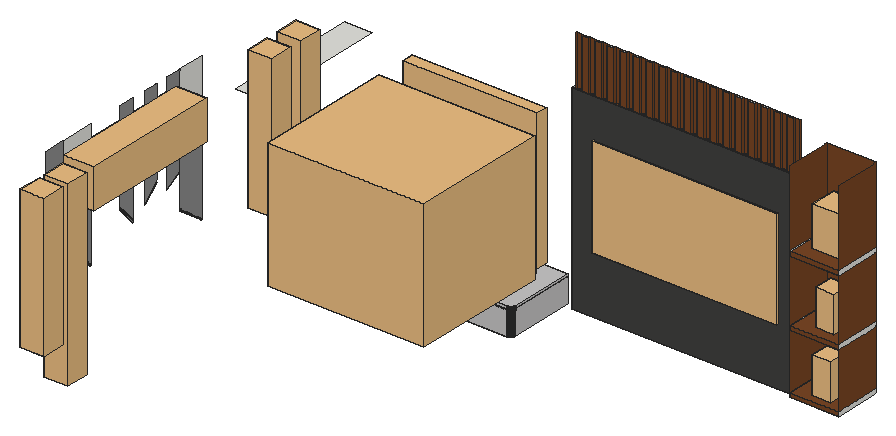
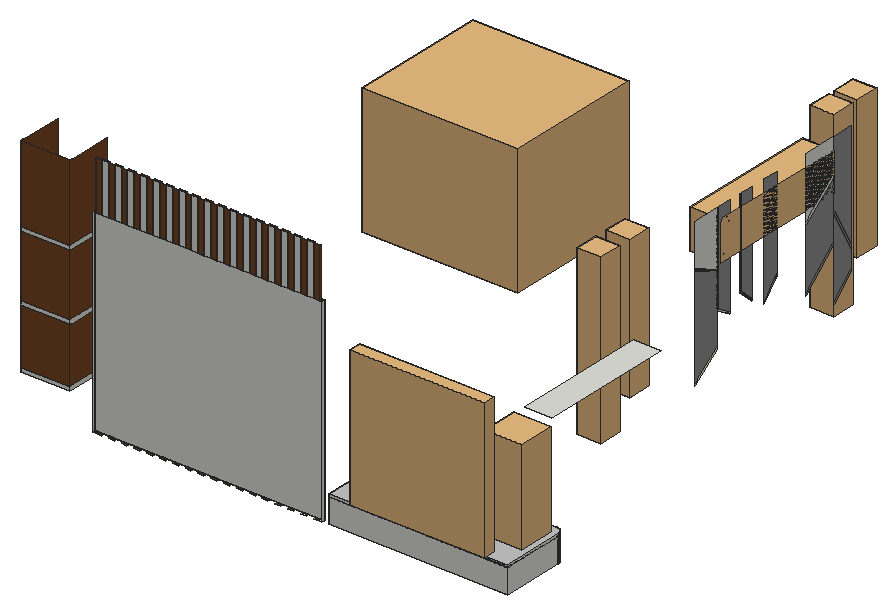
# SketchUp Ruby script. Lengths in inches.
U = 1.inch
M = Sketchup.active_model
def pt(a) = Geom::Point3d.new(a.map { |v| v * U })
def face(e, loops, mat)
  f = e.add_face(loops[0].map { |a| pt(a) })
  loops[1..].each { |l| e.add_face(l.map { |a| pt(a) }).erase! }
  f.material = f.back_material = mat if mat
  f
end
# faces: each face lists its corners as indices into pts; further lists are holes
def faces(e, pts, list, mat = nil) = list.each { |f| face(e, (f[0].is_a?(Array) ? f : [f]).map { |l| l.map { |i| pts[i] } }, mat) }
# xy, xz, yz: faces in a plane at the given z, y or x. An outline is a flat list of corners, or four numbers for a rectangle; further outlines are holes
def ring(l) = l.size == 4 ? [[l[0], l[1]], [l[2], l[1]], [l[2], l[3]], [l[0], l[3]]] : l.each_slice(2).to_a
def flat(e, list, mat, &to3) = list.each { |f| face(e, (f[0].is_a?(Array) ? f : [f]).map { |l| ring(l).map { |u, v| to3.(u, v) } }, mat) }
def xy(e, z, list, mat = nil) = flat(e, list, mat) { |x, y| [x, y, z] }
def xz(e, y, list, mat = nil) = flat(e, list, mat) { |x, z| [x, y, z] }
def yz(e, x, list, mat = nil) = flat(e, list, mat) { |y, z| [x, y, z] }
def lines(e, pts, list) = list.each { |a, b| e.add_line(pt(pts[a]), pt(pts[b])) }
# prism: a flat outline (further loops are holes) pulled along v
def prism(e, loops, v, mat = nil)
  f = face(e, loops, mat); d = Geom::Vector3d.new(v.map { |x| x * U })
  f.pushpull(f.normal.samedirection?(d) ? d.length : -d.length)
end
def box(e, o, s, mat = nil) = prism(e, [[o, [o[0] + s[0], o[1], o[2]], [o[0] + s[0], o[1] + s[1], o[2]], [o[0], o[1] + s[1], o[2]]]], [0, 0, s[2]], mat)
def at(x, y, z, deg = 0) = Geom::Transformation.translation(pt([x, y, z])) * Geom::Transformation.rotation(ORIGIN, Z_AXIS, deg.degrees)
def axes(o, x, y, z) = Geom::Transformation.new([*x, 0, *y, 0, *z, 0, *pt(o).to_a, 1])
def part(name) = M.definitions.add(name)
# library, detail: a bought-in or finely detailed component or shape, given as its bounding box
def library(name, o, s) = part(name).tap { |d| box(d.entities, o, s) }
def detail(e, o, s) = box(e.add_group.entities, o, s)
def put(e, d, t, mat = nil) = e.add_instance(d, t).tap { |i| i.material = mat if mat }
def group(e, t, mat = nil) = e.add_group.tap { |g| g.transformation = t; g.material = mat if mat }.entities
root = M.entities
M.materials.add("Emissive").color = [234, 236, 196]
M.materials.add("Generic").color = [198, 197, 197]
M.materials.add("Gold 10k").color = [251, 232, 180]
M.materials.add("Magma Rock Solid 19-50 100cm").color = [65, 65, 64]
M.materials.add("[Color M04]").color = [142, 142, 142]
M.materials.add("[Wood Veneer 01]").color = [120, 70, 37]
c1 = library("Lady Jane Collar",[-41.56,-7.87,0],[83.12,15.74,85.88])
c2 = library("Flowering Tree Twigs 63-18",[-6.76,-5.61,0],[12.33,12.14,31.28])
c3 = library("Milk Jug 92-17",[-1.54,-2.02,0],[3.08,4.6,8.29])
c4 = library("Vase Gerbera 18",[-3.31,-2.98,0],[6.3,6.31,11.9375])
c5 = library("Flat screen television",[0,1.41,1.14],[35.92,0.28,20.21])
c6 = library("Pendant 114-23",[-3.9375,-3.9375,-46.79],[7.875,7.875,46.79])
c7 = library("Milk Jug 92-23",[-3.1,-3.1,0],[6.18,6.2,11.88])
c8 = library("CUONGCV (3)",[45.61,64.16,23.25],[51.6,45.8,42.59])
c9 = library("Calla Lilies 63-10",[-4.34,-4.49,0],[8.67,8.83,13.09])
c10 = library("Streamline AC Unit ",[11.33,77.43,-2],[10.25,46.46,12.99])
xy(root,38.375,[[17.14,344.6875,16.8,344.71,16.46,344.78,16.13,344.89,15.82,345.04,15.53,345.23,15.27,345.46,15.05,345.72,14.85,346.01,14.7,346.32,14.59,346.64,14.52,346.98,14.5,347.33,14.5,367.875,73.93,367.875,73.93,346.37,73.91,346.15,73.87,345.93,73.8,345.72,73.7,345.53,73.58,345.34,73.43,345.18,73.27,345.03,73.09,344.91,72.89,344.82,72.68,344.74,72.47,344.7,72.25,344.6875],[150.92,366.625,151.83,367],[76.01,367.25,76.95,367.875],[76.95,367.25,78.89,367.875],[81.19,367.25,83.125,367.875],
  [150.92,367.25,151.83,367.875]])
xy(root,38.375,[[76.01,366.625,150.92,367]],"Magma Rock Solid 19-50 100cm")
xy(root,38.375,[[150.92,367,151.58,367.25],[85.43,367.25,87.36,367.875],[89.67,367.25,91.6,367.875],[93.9,367.25,95.84,367.875],[98.14,367.25,100.07,367.875],
  [102.38,367.25,104.3125,367.875],[106.62,367.25,108.55,367.875],[110.85,367.25,112.79,367.875],[115.09,367.25,117.02,367.875],[119.33,367.25,121.26,367.875],
  [123.57,367.25,125.5,367.875],[127.8,367.25,129.74,367.875],[132.04,367.25,133.97,367.875],[136.28,367.25,138.21,367.875],[140.52,367.25,142.45,367.875],
  [144.75,367.25,146.6875,367.875],[148.99,367.25,150.92,367.875]],"[Wood Veneer 01]")
xy(root,38.625,[[76.26,367,150.92,367.25]],"Emissive")
xy(root,46.375,[[17.14,344.6875,16.8,344.71,16.46,344.78,16.13,344.89,15.82,345.04,15.53,345.23,15.27,345.46,15.05,345.72,14.85,346.01,14.7,346.32,14.59,346.64,14.52,346.98,14.5,347.33,14.5,367.875,73.93,367.875,73.93,346.37,73.91,346.15,73.87,345.93,73.8,345.72,73.7,345.53,73.58,345.34,73.43,345.18,73.27,345.03,73.09,344.91,72.89,344.82,72.68,344.74,72.47,344.7,72.25,344.6875]])
xy(root,46.625,[[17.14,344.6875,16.8,344.71,16.46,344.78,16.13,344.89,15.82,345.04,15.53,345.23,15.27,345.46,15.05,345.72,14.85,346.01,14.7,346.32,14.59,346.64,14.52,346.98,14.5,347.33,14.5,367.875,73.93,367.875,73.93,346.37,73.91,346.15,73.87,345.93,73.8,345.72,73.7,345.53,73.58,345.34,73.43,345.18,73.27,345.03,73.09,344.91,72.89,344.82,72.68,344.74,72.47,344.7,72.25,344.6875]])
xy(root,47.375,[[17.14,344.6875,72.25,344.6875,72.47,344.7,72.68,344.74,72.89,344.82,73.09,344.91,73.27,345.03,73.43,345.18,73.58,345.34,73.7,345.53,73.8,345.72,73.87,345.93,73.91,346.15,73.93,346.37,73.93,367.875,14.5,367.875,14.5,347.33,14.52,346.98,14.59,346.64,14.7,346.32,14.85,346.01,15.05,345.72,15.27,345.46,15.53,345.23,15.82,345.04,16.13,344.89,16.46,344.78,16.8,344.71]],"Generic")
xy(root,47.59,[[159.58,352.5625,175.89,366.875]],"[Wood Veneer 01]")
xy(root,47.84,[[159.58,366.875,175.89,367.875]],"Emissive")
xy(root,48.99,[[159.58,352.5625,175.89,367.875]],"[Wood Veneer 01]")
xy(root,67.4,[[159.58,352.5625,175.89,366.875]],"[Wood Veneer 01]")
xy(root,67.65,[[159.58,366.875,175.89,367.875]],"Emissive")
xy(root,68.8,[[159.58,352.5625,175.89,367.875]],"[Wood Veneer 01]")
xy(root,89.4,[[159.58,352.5625,175.89,366.875]],"[Wood Veneer 01]")
xy(root,89.65,[[159.58,366.875,175.89,367.875]],"Emissive")
xy(root,90.8,[[159.58,352.5625,175.89,367.875]],"[Wood Veneer 01]")
xy(root,96,[[0,322.76,9,367.875]])
xy(root,103.375,[[76.26,367,151.58,367.25]],"Emissive")
xy(root,103.625,[[76.01,367.25,76.95,367.875],[78.89,367.25,81.19,367.875],[83.125,367.25,85.43,367.875],[87.36,367.25,89.67,367.875],[91.6,367.25,93.9,367.875],
  [95.84,367.25,98.14,367.875],[100.07,367.25,102.38,367.875],[104.3125,367.25,106.62,367.875],[108.55,367.25,110.85,367.875],[112.79,367.25,115.09,367.875],
  [117.02,367.25,119.33,367.875],[121.26,367.25,123.57,367.875],[125.5,367.25,127.8,367.875],[129.74,367.25,132.04,367.875],[133.97,367.25,136.28,367.875],
  [138.21,367.25,140.52,367.875],[142.45,367.25,144.75,367.875],[146.6875,367.25,148.99,367.875],[150.92,367.25,151.83,367.875]])
xy(root,103.625,[[76.01,366.625,151.83,367]],"Magma Rock Solid 19-50 100cm")
xy(root,103.625,[[76.95,367.25,78.89,367.875],[81.19,367.25,83.125,367.875],[85.43,367.25,87.36,367.875],[89.67,367.25,91.6,367.875],[93.9,367.25,95.84,367.875],
  [98.14,367.25,100.07,367.875],[102.38,367.25,104.3125,367.875],[106.62,367.25,108.55,367.875],[110.85,367.25,112.79,367.875],[115.09,367.25,117.02,367.875],
  [119.33,367.25,121.26,367.875],[123.57,367.25,125.5,367.875],[127.8,367.25,129.74,367.875],[132.04,367.25,133.97,367.875],[136.28,367.25,138.21,367.875],
  [140.52,367.25,142.45,367.875],[144.75,367.25,146.6875,367.875],[148.99,367.25,150.92,367.875]],"[Wood Veneer 01]")
xz(root,240.18,[[8.9375,70.9375,9,97.25],[8.9375,98.25,9,120]])
xz(root,240.43,[[8.9375,88.44,9,107.62]],"[Color M04]")
xz(root,251.56,[[8.9375,99.77,9,120]])
xz(root,251.56,[[8.9375,78.66,9,99.01]],"[Color M04]")
xz(root,263.87,[[8.9375,89.91,9,120]])
xz(root,268.93,[[8.9375,83.81,9,120]],"[Color M04]")
xz(root,274.12,[[8.9375,86.8125,9,120]],"[Color M04]")
xz(root,278.81,[[8.9375,91.37,9,120]],"[Color M04]")
xz(root,283.12,[[8.9375,87,9,120]],"[Color M04]")
xz(root,288.31,[[8.9375,90.1,9,120]],"[Color M04]")
xz(root,288.56,[[8.9375,101.89,9,120]])
xz(root,288.56,[[8.9375,78.64,9,101.51]],"[Color M04]")
xz(root,344.6875,[[17.14,38.375,44.69,46.375],[45.09,38.375,72.25,46.375],[17.14,46.625,72.25,47.375]],"Generic")
xz(root,344.6875,[[44.69,38.375,45.09,46.375],[17.14,46.375,72.25,46.625]],"Gold 10k")
xz(root,352.5625,[[159.58,47.59,175.89,48.99],[159.58,67.4,175.89,68.8],[159.58,89.4,175.89,90.8]],"[Wood Veneer 01]")
xz(root,366.625,[[76.01,38.375,151.83,103.625]],"Magma Rock Solid 19-50 100cm")
xz(root,366.875,[[159.58,47.59,175.89,47.84],[159.58,67.4,175.89,67.65],[159.58,89.4,175.89,89.4375],[159.58,89.4375,175.89,89.65]],"Emissive")
xz(root,367,[[150.92,38.375,150.92,38.625,76.26,38.625,76.26,103.375,151.58,103.375,151.58,38.375]])
xz(root,367,[[76.01,38.375,150.92,38.625],[151.58,38.375,151.83,103.625],[76.01,38.625,76.26,103.375],[76.01,103.375,151.58,103.625]],"Emissive")
xz(root,367.25,[[150.92,38.375,150.92,38.625,76.26,38.625,76.26,103.375,151.58,103.375,151.58,38.375]])
xz(root,367.25,[[76.01,38.375,76.95,38.625],[76.95,38.375,78.89,38.625],[81.19,38.375,83.125,38.625],[85.43,38.375,87.36,38.625],[89.67,38.375,91.6,38.625],
  [93.9,38.375,95.84,38.625],[98.14,38.375,100.07,38.625],[102.38,38.375,104.3125,38.625],[106.62,38.375,108.55,38.625],[110.85,38.375,112.79,38.625],
  [115.09,38.375,117.02,38.625],[119.33,38.375,121.26,38.625],[123.57,38.375,125.5,38.625],[127.8,38.375,129.74,38.625],[132.04,38.375,133.97,38.625],
  [136.28,38.375,138.21,38.625],[140.52,38.375,142.45,38.625],[144.75,38.375,146.6875,38.625],[148.99,38.375,150.92,38.625],[151.58,38.375,151.83,103.625],
  [76.01,38.625,76.26,103.375],[76.01,103.375,76.95,103.625],[76.95,103.375,78.89,103.625],[78.89,103.375,81.19,103.625],[81.19,103.375,83.125,103.625],
  [83.125,103.375,85.43,103.625],[85.43,103.375,87.36,103.625],[87.36,103.375,89.67,103.625],[89.67,103.375,91.6,103.625],[91.6,103.375,93.9,103.625],
  [93.9,103.375,95.84,103.625],[95.84,103.375,98.14,103.625],[98.14,103.375,100.07,103.625],[100.07,103.375,102.38,103.625],[102.38,103.375,104.3125,103.625],
  [104.3125,103.375,106.62,103.625],[106.62,103.375,108.55,103.625],[108.55,103.375,110.85,103.625],[110.85,103.375,112.79,103.625],[112.79,103.375,115.09,103.625],
  [115.09,103.375,117.02,103.625],[117.02,103.375,119.33,103.625],[119.33,103.375,121.26,103.625],[121.26,103.375,123.57,103.625],[123.57,103.375,125.5,103.625],
  [125.5,103.375,127.8,103.625],[127.8,103.375,129.74,103.625],[129.74,103.375,132.04,103.625],[132.04,103.375,133.97,103.625],[133.97,103.375,136.28,103.625],
  [136.28,103.375,138.21,103.625],[138.21,103.375,140.52,103.625],[140.52,103.375,142.45,103.625],[142.45,103.375,144.75,103.625],[144.75,103.375,146.6875,103.625],
  [146.6875,103.375,148.99,103.625],[148.99,103.375,150.92,103.625],[150.92,103.375,151.58,103.625]],"Emissive")
xz(root,367.25,[[78.89,103.625,81.19,120],[83.125,103.625,85.43,120],[87.36,103.625,89.67,120],[91.6,103.625,93.9,120],[95.84,103.625,98.14,120],
  [100.07,103.625,102.38,120],[104.3125,103.625,106.62,120],[108.55,103.625,110.85,120],[112.79,103.625,115.09,120],[117.02,103.625,119.33,120],
  [121.26,103.625,123.57,120],[125.5,103.625,127.8,120],[129.74,103.625,132.04,120],[133.97,103.625,136.28,120],[138.21,103.625,140.52,120],
  [142.45,103.625,144.75,120],[146.6875,103.625,148.99,120]],"[Wood Veneer 01]")
xz(root,367.875,[[14.5,38.375,73.93,46.375],[14.5,46.375,73.93,46.625],[14.5,46.625,73.93,47.375],[159.58,47.84,175.89,48.99],[159.58,67.65,175.89,68.8],
  [159.58,89.65,175.89,90.8],[78.89,103.625,81.19,120],[83.125,103.625,85.43,120],[87.36,103.625,89.67,120],[91.6,103.625,93.9,120],
  [95.84,103.625,98.14,120],[100.07,103.625,102.38,120],[104.3125,103.625,106.62,120],[108.55,103.625,110.85,120],[112.79,103.625,115.09,120],
  [117.02,103.625,119.33,120],[121.26,103.625,123.57,120],[125.5,103.625,127.8,120],[129.74,103.625,132.04,120],[133.97,103.625,136.28,120],
  [138.21,103.625,140.52,120],[142.45,103.625,144.75,120],[146.6875,103.625,148.99,120]])
xz(root,367.875,[[159.58,48.99,175.89,67.65],[159.58,68.8,175.89,89.65],[159.58,90.8,175.89,116.25],[76.95,103.625,78.89,120],[81.19,103.625,83.125,120],
  [85.43,103.625,87.36,120],[89.67,103.625,91.6,120],[93.9,103.625,95.84,120],[98.14,103.625,100.07,120],[102.38,103.625,104.3125,120],
  [106.62,103.625,108.55,120],[110.85,103.625,112.79,120],[115.09,103.625,117.02,120],[119.33,103.625,121.26,120],[123.57,103.625,125.5,120],
  [127.8,103.625,129.74,120],[132.04,103.625,133.97,120],[136.28,103.625,138.21,120],[140.52,103.625,142.45,120],[144.75,103.625,146.6875,120],
  [148.99,103.625,150.92,120]],"[Wood Veneer 01]")
yz(root,8.9375,[[251.56,99.01,251.56,99.77,240.43,108.38,240.43,107.62]])
yz(root,8.9375,[[297.48,71.32,297.48,71.82,288.56,78.64,288.56,78.14],[283.12,86.5,288.31,89.6,288.31,90.1,283.12,87],[288.56,101.51,297.48,105.77,297.48,106.14,288.56,101.89]],"Emissive")
yz(root,8.9375,[[240.18,70.25,240.18,70.9375,233,77.53,233,76.84],[251.56,77.93,251.56,78.66,240.43,88.44,240.43,87.71],[268.93,83.18,268.93,83.81,263.87,89.91,263.87,89.29],[233,83.85,240.18,97.25,240.18,98.25,233,84.85],[274.12,86.125,278.81,90.68,278.81,91.37,274.12,86.8125]],"[Color M04]")
yz(root,9,[[251.56,99.77,251.56,120,240.43,120,240.43,108.38],[288.56,101.89,297.48,106.14,297.48,120,288.56,120]])
yz(root,9,[[240.18,70.9375,240.18,97.25,233,83.85,233,77.53],[297.48,71.82,297.48,105.77,288.56,101.51,288.56,78.64],[251.56,78.66,251.56,99.01,240.43,107.62,240.43,88.44],[268.93,83.81,268.93,120,263.87,120,263.87,89.91],[233,84.85,240.18,98.25,240.18,120,233,120],
  [274.12,86.8125,278.81,91.37,278.81,120,274.12,120],[283.12,87,288.31,90.1,288.31,120,283.12,120]],"[Color M04]")
yz(root,14.5,[[347.33,38.375,367.875,46.375],[347.33,46.375,367.875,46.625],[347.33,46.625,367.875,47.375]])
yz(root,73.93,[[346.37,38.375,367.875,46.375],[346.37,46.625,367.875,47.375]],"Generic")
yz(root,73.93,[[346.37,46.375,367.875,46.625]],"Gold 10k")
yz(root,76.01,[[367.25,38.375,367.875,103.625]])
yz(root,76.01,[[366.625,38.375,367,103.625]],"Magma Rock Solid 19-50 100cm")
yz(root,76.26,[[367,38.625,367.25,103.375]],"Emissive")
yz(root,76.95,[[367.25,103.625,367.875,120]],"[Wood Veneer 01]")
yz(root,78.89,[[367.25,103.625,367.875,120]],"[Wood Veneer 01]")
yz(root,81.19,[[367.25,103.625,367.875,120]],"[Wood Veneer 01]")
yz(root,83.125,[[367.25,103.625,367.875,120]],"[Wood Veneer 01]")
yz(root,85.43,[[367.25,103.625,367.875,120]],"[Wood Veneer 01]")
yz(root,87.36,[[367.25,103.625,367.875,120]],"[Wood Veneer 01]")
yz(root,89.67,[[367.25,103.625,367.875,120]],"[Wood Veneer 01]")
yz(root,91.6,[[367.25,103.625,367.875,120]],"[Wood Veneer 01]")
yz(root,93.9,[[367.25,103.625,367.875,120]],"[Wood Veneer 01]")
yz(root,95.84,[[367.25,103.625,367.875,120]],"[Wood Veneer 01]")
yz(root,98.14,[[367.25,103.625,367.875,120]],"[Wood Veneer 01]")
yz(root,100.07,[[367.25,103.625,367.875,120]],"[Wood Veneer 01]")
yz(root,102.38,[[367.25,103.625,367.875,120]],"[Wood Veneer 01]")
yz(root,104.3125,[[367.25,103.625,367.875,120]],"[Wood Veneer 01]")
yz(root,106.62,[[367.25,103.625,367.875,120]],"[Wood Veneer 01]")
yz(root,108.55,[[367.25,103.625,367.875,120]],"[Wood Veneer 01]")
yz(root,110.85,[[367.25,103.625,367.875,120]],"[Wood Veneer 01]")
yz(root,112.79,[[367.25,103.625,367.875,120]],"[Wood Veneer 01]")
yz(root,115.09,[[367.25,103.625,367.875,120]],"[Wood Veneer 01]")
yz(root,117.02,[[367.25,103.625,367.875,120]],"[Wood Veneer 01]")
yz(root,119.33,[[367.25,103.625,367.875,120]],"[Wood Veneer 01]")
yz(root,121.26,[[367.25,103.625,367.875,120]],"[Wood Veneer 01]")
yz(root,123.57,[[367.25,103.625,367.875,120]],"[Wood Veneer 01]")
yz(root,125.5,[[367.25,103.625,367.875,120]],"[Wood Veneer 01]")
yz(root,127.8,[[367.25,103.625,367.875,120]],"[Wood Veneer 01]")
yz(root,129.74,[[367.25,103.625,367.875,120]],"[Wood Veneer 01]")
yz(root,132.04,[[367.25,103.625,367.875,120]],"[Wood Veneer 01]")
yz(root,133.97,[[367.25,103.625,367.875,120]],"[Wood Veneer 01]")
yz(root,136.28,[[367.25,103.625,367.875,120]],"[Wood Veneer 01]")
yz(root,138.21,[[367.25,103.625,367.875,120]],"[Wood Veneer 01]")
yz(root,140.52,[[367.25,103.625,367.875,120]],"[Wood Veneer 01]")
yz(root,142.45,[[367.25,103.625,367.875,120]],"[Wood Veneer 01]")
yz(root,144.75,[[367.25,103.625,367.875,120]],"[Wood Veneer 01]")
yz(root,146.6875,[[367.25,103.625,367.875,120]],"[Wood Veneer 01]")
yz(root,148.99,[[367.25,103.625,367.875,120]],"[Wood Veneer 01]")
yz(root,150.92,[[367,38.375,367.25,38.625]],"Emissive")
yz(root,150.92,[[367.25,103.625,367.875,120]],"[Wood Veneer 01]")
yz(root,151.58,[[367,38.375,367.25,103.375]],"Emissive")
yz(root,151.83,[[367.25,38.375,367.875,103.625]])
yz(root,151.83,[[366.625,38.375,367,103.625]],"Magma Rock Solid 19-50 100cm")
yz(root,159.58,[[352.5625,47.59,366.875,47.59,366.875,47.84,367.875,47.84,367.875,48.99,352.5625,48.99],[352.5625,67.4,366.875,67.4,366.875,67.65,367.875,67.65,367.875,68.8,352.5625,68.8],[352.5625,89.4,366.875,89.4,366.875,89.65,367.875,89.65,367.875,90.8,352.5625,90.8]])
yz(root,159.58,[[352.5625,48.99,367.875,48.99,367.875,67.65,366.875,67.65,366.875,67.4,352.5625,67.4],[352.5625,68.8,367.875,68.8,367.875,89.65,366.875,89.65,366.875,89.4,352.5625,89.4],[352.5625,90.8,367.875,90.8,367.875,116.25,366.875,116.25,366.875,116,352.5625,116]],"[Wood Veneer 01]")
yz(root,175.89,[[352.5625,47.59,352.5625,48.99,367.875,48.99,367.875,47.84,366.875,47.84,366.875,47.59],[352.5625,67.4,352.5625,68.8,367.875,68.8,367.875,67.65,366.875,67.65,366.875,67.4],[352.5625,89.4,352.5625,90.8,367.875,90.8,367.875,89.65,366.875,89.65,366.875,89.4]])
yz(root,175.89,[[352.5625,48.99,352.5625,67.4,366.875,67.4,366.875,67.65,367.875,67.65,367.875,48.99],[352.5625,68.8,352.5625,89.4,366.875,89.4,366.875,89.65,367.875,89.65,367.875,68.8],[352.5625,90.8,352.5625,116,366.875,116,366.875,116.25,367.875,116.25,367.875,90.8]],"[Wood Veneer 01]")
p = [[16.8,344.71,38.375],[16.8,344.71,46.375],[16.46,344.78,46.375],[16.46,344.78,38.375],[17.14,344.6875,38.375],[17.14,344.6875,46.375],
  [72.47,344.7,38.375],[72.47,344.7,46.375],[72.25,344.6875,46.375],[72.25,344.6875,38.375],[72.68,344.74,38.375],[72.68,344.74,46.375],
  [72.89,344.82,38.375],[72.89,344.82,46.375],[16.13,344.89,46.375],[16.13,344.89,38.375],[73.09,344.91,38.375],[73.09,344.91,46.375],
  [15.82,345.04,46.375],[15.82,345.04,38.375],[73.27,345.03,38.375],[73.27,345.03,46.375],[15.53,345.23,46.375],[15.53,345.23,38.375],
  [73.43,345.18,38.375],[73.43,345.18,46.375],[15.27,345.46,46.375],[15.27,345.46,38.375],[73.58,345.34,38.375],[73.58,345.34,46.375],
  [73.7,345.53,38.375],[73.7,345.53,46.375],[15.05,345.72,46.375],[15.05,345.72,38.375],[73.8,345.72,38.375],[73.8,345.72,46.375],
  [14.85,346.01,46.375],[14.85,346.01,38.375],[73.87,345.93,38.375],[73.87,345.93,46.375],[73.91,346.15,38.375],[73.91,346.15,46.375],
  [14.7,346.32,46.375],[14.7,346.32,38.375],[73.93,346.37,38.375],[73.93,346.37,46.375],[14.59,346.64,46.375],[14.59,346.64,38.375],
  [14.52,346.98,46.375],[14.52,346.98,38.375],[14.5,347.33,46.375],[14.5,347.33,38.375],[16.46,344.78,46.625],[16.8,344.71,46.625],
  [17.14,344.6875,46.625],[72.25,344.6875,46.625],[72.47,344.7,46.625],[72.68,344.74,46.625],[72.89,344.82,46.625],[16.13,344.89,46.625],
  [73.09,344.91,46.625],[15.82,345.04,46.625],[73.27,345.03,46.625],[15.53,345.23,46.625],[73.43,345.18,46.625],[15.27,345.46,46.625],
  [73.58,345.34,46.625],[73.7,345.53,46.625],[15.05,345.72,46.625],[73.8,345.72,46.625],[14.85,346.01,46.625],[73.87,345.93,46.625],
  [73.91,346.15,46.625],[14.7,346.32,46.625],[73.93,346.37,46.625],[14.59,346.64,46.625],[14.52,346.98,46.625],[14.5,347.33,46.625],
  [16.8,344.71,47.375],[16.46,344.78,47.375],[17.14,344.6875,47.375],[72.47,344.7,47.375],[72.25,344.6875,47.375],[72.68,344.74,47.375],
  [72.89,344.82,47.375],[16.13,344.89,47.375],[73.09,344.91,47.375],[15.82,345.04,47.375],[73.27,345.03,47.375],[15.53,345.23,47.375],
  [73.43,345.18,47.375],[15.27,345.46,47.375],[73.58,345.34,47.375],[73.7,345.53,47.375],[15.05,345.72,47.375],[73.8,345.72,47.375],
  [14.85,346.01,47.375],[73.87,345.93,47.375],[73.91,346.15,47.375],[14.7,346.32,47.375],[73.93,346.37,47.375],[14.59,346.64,47.375],
  [14.52,346.98,47.375],[14.5,347.33,47.375],[9,233,76.84],[9,240.18,70.25],[8.9375,240.18,70.25],[8.9375,233,76.84],
  [9,240.18,70.9375],[9,233,77.53],[8.9375,233,77.53],[8.9375,240.18,70.9375],[9,288.56,78.14],[9,297.48,71.32],
  [8.9375,297.48,71.32],[8.9375,288.56,78.14],[9,297.48,71.82],[9,288.56,78.64],[8.9375,288.56,78.64],[8.9375,297.48,71.82],
  [9,240.43,87.71],[9,251.56,77.93],[8.9375,251.56,77.93],[8.9375,240.43,87.71],[9,251.56,78.66],[9,240.43,88.44],
  [8.9375,240.43,88.44],[8.9375,251.56,78.66],[9,263.87,89.29],[9,268.93,83.18],[8.9375,268.93,83.18],[8.9375,263.87,89.29],
  [9,233,83.85],[9,240.18,97.25],[8.9375,240.18,97.25],[8.9375,233,83.85],[9,268.93,83.81],[9,263.87,89.91],
  [8.9375,263.87,89.91],[8.9375,268.93,83.81],[9,240.18,98.25],[9,233,84.85],[8.9375,233,84.85],[8.9375,240.18,98.25],
  [9,274.12,86.125],[9,278.81,90.68],[8.9375,278.81,90.68],[8.9375,274.12,86.125],[9,283.12,86.5],[9,288.31,89.6],
  [8.9375,288.31,89.6],[8.9375,283.12,86.5],[9,278.81,91.37],[9,274.12,86.8125],[8.9375,274.12,86.8125],[8.9375,278.81,91.37],
  [9,288.31,90.1],[9,283.12,87],[8.9375,283.12,87],[8.9375,288.31,90.1],[9,240.43,107.62],[9,251.56,99.01],
  [8.9375,251.56,99.01],[8.9375,240.43,107.62],[9,251.56,99.77],[9,240.43,108.38],[8.9375,240.43,108.38],[8.9375,251.56,99.77],
  [9,288.56,101.51],[9,297.48,105.77],[8.9375,297.48,105.77],[8.9375,288.56,101.51],[9,297.48,106.14],[9,288.56,101.89],
  [8.9375,288.56,101.89],[8.9375,297.48,106.14]]
faces(root,p,[[0,1,2,3],[4,5,1,0],[3,2,14,15],[15,14,18,19],[19,18,22,23],[23,22,26,27],[27,26,32,33],[33,32,36,37],
  [37,36,42,43],[43,42,46,47],[47,46,48,49],[49,48,50,51],[78,79,52,53],[80,78,53,54],[79,85,59,52],[85,87,61,59],
  [87,89,63,61],[89,91,65,63],[91,94,68,65],[94,96,70,68],[96,99,73,70],[99,101,75,73],[101,102,76,75],[102,103,77,76],
  [104,105,106,107],[108,109,110,111],[140,141,142,143],[152,153,154,155],[160,161,162,163]])
faces(root,p,[[6,7,8,9],[10,11,7,6],[12,13,11,10],[16,17,13,12],[20,21,17,16],[24,25,21,20],[28,29,25,24],[30,31,29,28],
  [34,35,31,30],[38,39,35,34],[40,41,39,38],[44,45,41,40],[81,82,55,56],[83,81,56,57],[84,83,57,58],[86,84,58,60],
  [88,86,60,62],[90,88,62,64],[92,90,64,66],[93,92,66,67],[95,93,67,69],[97,95,69,71],[98,97,71,72],[100,98,72,74]],"Generic")
faces(root,p,[[52,2,1,53],[53,1,5,54],[55,8,7,56],[56,7,11,57],[57,11,13,58],[59,14,2,52],[58,13,17,60],[61,18,14,59],
  [60,17,21,62],[63,22,18,61],[62,21,25,64],[65,26,22,63],[64,25,29,66],[66,29,31,67],[68,32,26,65],[67,31,35,69],
  [70,36,32,68],[69,35,39,71],[71,39,41,72],[73,42,36,70],[72,41,45,74],[75,46,42,73],[76,48,46,75],[77,50,48,76]],"Gold 10k")
faces(root,p,[[112,113,114,115],[116,117,118,119],[120,121,122,123],[124,125,126,127],[128,129,130,131],[136,137,138,139],[148,149,150,151],[156,157,158,159],
  [164,165,166,167],[168,169,170,171],[172,173,174,175]],"Emissive")
faces(root,p,[[132,133,134,135],[144,145,146,147]],"[Color M04]")
put(root,c1,axes([43.76,366.95,47.375],[-0.53578,0,0],[0,-0.25182,0],[0,0,0.53578]))
put(root,c2,at(23.24,353.18,47.375))
put(root,c3,at(66,360.01,47.375))
put(root,c4,at(168.17,357.92,48.99))
put(root,c5,axes([83.35,362.46,55.99],[1.69858,0,0],[0,2.47,0],[0,0,1.62851]))
put(root,c6,axes([20.25,227.07,120],[1,0,0],[0,1,0],[0,0,1.28]))
put(root,c6,axes([20.25,323.49,120],[1,0,0],[0,1,0],[0,0,1.18]))
put(root,c7,at(168.34,359.14,68.8))
put(root,c6,at(20.25,217.32,120))
put(root,c6,at(20.25,311.49,120))
put(root,c8,at(14.11,197.32,62.16))
put(root,c9,at(167.34,361.93,90.8))
put(root,c10,at(30.58,364.07,104.91,180))
